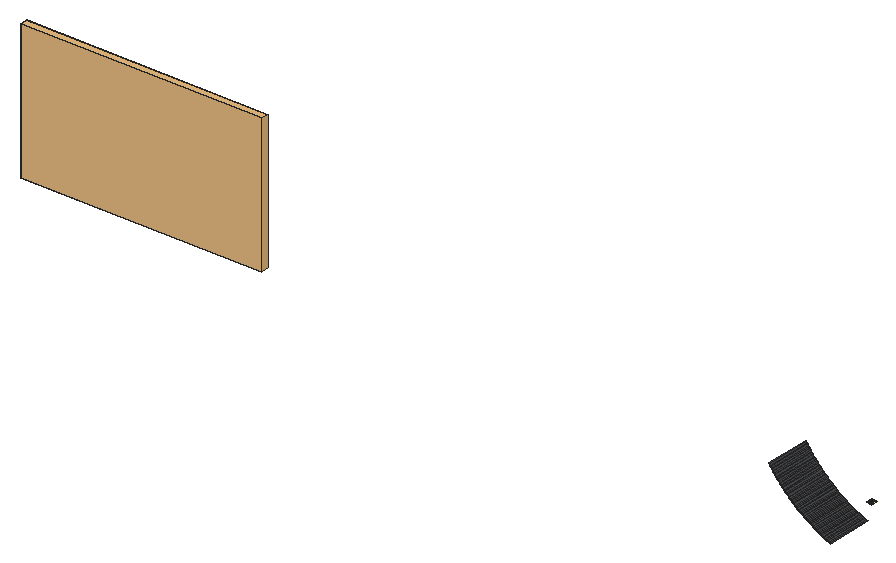
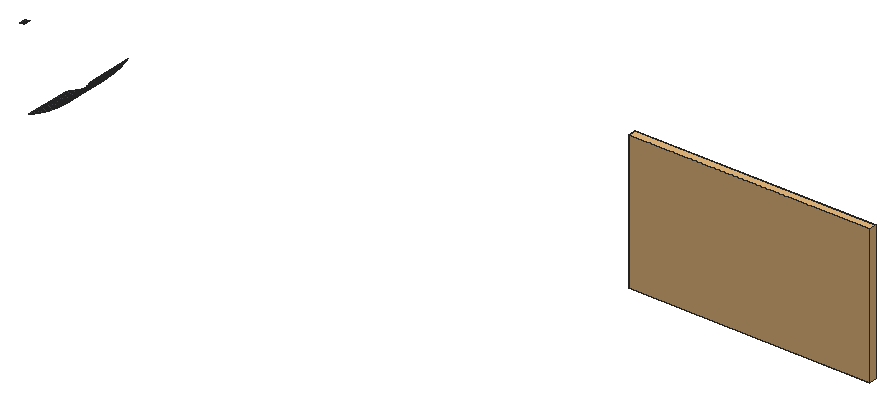
# SketchUp Ruby script. Lengths in inches.
U = 1.inch
M = Sketchup.active_model
def pt(a) = Geom::Point3d.new(a.map { |v| v * U })
def face(e, loops, mat)
  f = e.add_face(loops[0].map { |a| pt(a) })
  loops[1..].each { |l| e.add_face(l.map { |a| pt(a) }).erase! }
  f.material = f.back_material = mat if mat
  f
end
# faces: each face lists its corners as indices into pts; further lists are holes
def faces(e, pts, list, mat = nil) = list.each { |f| face(e, (f[0].is_a?(Array) ? f : [f]).map { |l| l.map { |i| pts[i] } }, mat) }
# xy, xz, yz: faces in a plane at the given z, y or x. An outline is a flat list of corners, or four numbers for a rectangle; further outlines are holes
def ring(l) = l.size == 4 ? [[l[0], l[1]], [l[2], l[1]], [l[2], l[3]], [l[0], l[3]]] : l.each_slice(2).to_a
def flat(e, list, mat, &to3) = list.each { |f| face(e, (f[0].is_a?(Array) ? f : [f]).map { |l| ring(l).map { |u, v| to3.(u, v) } }, mat) }
def xy(e, z, list, mat = nil) = flat(e, list, mat) { |x, y| [x, y, z] }
def xz(e, y, list, mat = nil) = flat(e, list, mat) { |x, z| [x, y, z] }
def yz(e, x, list, mat = nil) = flat(e, list, mat) { |y, z| [x, y, z] }
def lines(e, pts, list) = list.each { |a, b| e.add_line(pt(pts[a]), pt(pts[b])) }
# prism: a flat outline (further loops are holes) pulled along v
def prism(e, loops, v, mat = nil)
  f = face(e, loops, mat); d = Geom::Vector3d.new(v.map { |x| x * U })
  f.pushpull(f.normal.samedirection?(d) ? d.length : -d.length)
end
def box(e, o, s, mat = nil) = prism(e, [[o, [o[0] + s[0], o[1], o[2]], [o[0] + s[0], o[1] + s[1], o[2]], [o[0], o[1] + s[1], o[2]]]], [0, 0, s[2]], mat)
def at(x, y, z, deg = 0) = Geom::Transformation.translation(pt([x, y, z])) * Geom::Transformation.rotation(ORIGIN, Z_AXIS, deg.degrees)
def axes(o, x, y, z) = Geom::Transformation.new([*x, 0, *y, 0, *z, 0, *pt(o).to_a, 1])
def part(name) = M.definitions.add(name)
# library, detail: a bought-in or finely detailed component or shape, given as its bounding box
def library(name, o, s) = part(name).tap { |d| box(d.entities, o, s) }
def detail(e, o, s) = box(e.add_group.entities, o, s)
def put(e, d, t, mat = nil) = e.add_instance(d, t).tap { |i| i.material = mat if mat }
def group(e, t, mat = nil) = e.add_group.tap { |g| g.transformation = t; g.material = mat if mat }.entities
root = M.entities
M.materials.add("1432 AP 8245 TAR ROAD").color = [71, 72, 75]
M.materials.add("Outer Light").color = [251, 217, 152]
M.materials.add("[Wood Cherry Original]").color = [152, 86, 42]
c1 = library("Group\#43",[0,-2,0],[63,2,36])
p = [[264.96,107.37,158.64],[265.22,107.37,158.53],[265.22,95.37,158.53],[264.96,95.37,158.64],[264.7,107.37,158.75],[264.7,95.37,158.75],
  [264.44,107.37,158.87],[264.44,95.37,158.87],[264.19,107.37,158.98],[264.19,95.37,158.98],[263.93,107.37,159.1],[263.93,95.37,159.1],
  [263.67,107.37,159.22],[263.67,95.37,159.22],[263.42,107.37,159.34],[263.42,95.37,159.34],[263.16,107.37,159.46],[263.16,95.37,159.46],
  [262.91,107.37,159.59],[262.91,95.37,159.59],[262.66,107.37,159.72],[262.66,95.37,159.72],[262.4,107.37,159.85],[262.4,95.37,159.85],
  [262.15,107.37,159.98],[262.15,95.37,159.98],[261.91,107.37,160.11],[261.91,95.37,160.11],[261.66,107.37,160.25],[261.66,95.37,160.25],
  [261.41,107.37,160.38],[261.41,95.37,160.38],[261.16,107.37,160.52],[261.16,95.37,160.52],[260.92,107.37,160.66],[260.92,95.37,160.66],
  [260.67,107.37,160.81],[260.67,95.37,160.81],[260.43,107.37,160.95],[260.43,95.37,160.95],[260.19,107.37,161.1],[260.19,95.37,161.1],
  [259.95,107.37,161.25],[259.95,95.37,161.25],[259.71,107.37,161.4],[259.71,95.37,161.4],[259.47,107.37,161.55],[259.47,95.37,161.55],
  [259.24,107.37,161.7],[259.24,95.37,161.7],[259,107.37,161.86],[259,95.37,161.86],[258.76,107.37,162.02],[258.76,95.37,162.02],
  [258.53,107.37,162.18],[258.53,95.37,162.18],[258.3,107.37,162.34],[258.3,95.37,162.34],[258.07,107.37,162.5],[258.07,95.37,162.5],
  [257.84,107.37,162.67],[257.84,95.37,162.67],[257.61,107.37,162.83],[257.61,95.37,162.83],[257.38,107.37,163],[257.38,95.37,163],
  [257.16,107.37,163.17],[257.16,95.37,163.17],[256.94,107.37,163.35],[256.94,95.37,163.35],[256.71,107.37,163.52],[256.71,95.37,163.52],
  [256.49,107.37,163.7],[256.49,95.37,163.7],[256.27,107.37,163.875],[256.27,95.37,163.875],[256.05,107.37,164.05],[256.05,95.37,164.05],
  [255.84,107.37,164.23],[255.84,95.37,164.23],[255.62,107.37,164.42],[255.62,95.37,164.42],[255.41,107.37,164.6],[255.41,95.37,164.6],
  [255.19,107.37,164.79],[255.19,95.37,164.79],[254.98,107.37,164.98],[254.98,95.37,164.98],[254.77,107.37,165.17],[254.77,95.37,165.17],
  [254.5625,107.37,165.36],[254.5625,95.37,165.36],[254.36,107.37,165.55],[254.36,95.37,165.55],[254.15,107.37,165.74],[254.15,95.37,165.74],
  [253.95,107.37,165.94],[253.95,95.37,165.94],[253.74,107.37,166.14],[253.74,95.37,166.14],[253.54,107.37,166.34],[253.54,95.37,166.34],
  [253.35,107.37,166.54],[253.35,95.37,166.54],[253.15,107.37,166.74],[253.15,95.37,166.74],[252.95,107.37,166.94],[252.95,95.37,166.94],
  [252.76,107.37,167.15],[252.76,95.37,167.15],[252.5625,107.37,167.36],[252.5625,95.37,167.36],[252.375,107.37,167.5625],[252.375,95.37,167.5625],
  [252.18,107.37,167.77],[252.18,95.37,167.77],[252,107.37,167.98],[252,95.37,167.98],[251.81,107.37,168.2],[251.81,95.37,168.2],
  [251.625,107.37,168.41],[251.625,95.37,168.41],[251.44,107.37,168.63],[251.44,95.37,168.63],[251.26,107.37,168.84],[251.26,95.37,168.84],
  [251.08,107.37,169.0625],[251.08,95.37,169.0625],[250.9,107.37,169.28],[250.9,95.37,169.28],[250.73,107.37,169.5],[250.73,95.37,169.5],
  [250.55,107.37,169.73],[250.55,95.37,169.73],[250.38,107.37,169.95],[250.38,95.37,169.95],[250.21,107.37,170.18],[250.21,95.37,170.18],
  [250.04,107.37,170.4],[250.04,95.37,170.4],[249.875,107.37,170.63],[249.875,95.37,170.63],[249.71,107.37,170.86],[249.71,95.37,170.86],
  [249.55,107.37,171.09],[249.55,95.37,171.09],[249.38,107.37,171.32],[249.38,95.37,171.32],[249.23,107.37,171.56],[249.23,95.37,171.56],
  [275.63,95.37,171.57],[275.79,95.37,171.54],[275.79,96.87,171.54],[275.63,96.87,171.57],[275.63,96.87,171.57],[275.79,96.87,171.54],
  [275.79,95.37,171.54],[275.63,95.37,171.57],[275.95,95.37,171.52],[275.95,96.87,171.52],[275.95,96.87,171.52],[275.95,95.37,171.52],
  [249.07,107.37,171.79],[249.07,95.37,171.79],[275.16,95.37,171.66],[275.32,95.37,171.625],[275.32,96.87,171.625],[275.16,96.87,171.66],
  [275.16,96.87,171.66],[275.32,96.87,171.625],[275.32,95.37,171.625],[275.16,95.37,171.66],[275.48,95.37,171.6],[275.48,96.87,171.6],
  [275.48,96.87,171.6],[275.48,95.37,171.6],[274.69,95.37,171.75],[274.84,95.37,171.72],[274.84,96.87,171.72],[274.69,96.87,171.75],
  [274.69,96.87,171.75],[274.84,96.87,171.72],[274.84,95.37,171.72],[274.69,95.37,171.75],[275,95.37,171.6875],[275,96.87,171.6875],
  [275,96.87,171.6875],[275,95.37,171.6875]]
faces(root,p,[[0,1,2,3],[4,0,3,5],[6,4,5,7],[8,6,7,9],[10,8,9,11],[12,10,11,13],[14,12,13,15],[16,14,15,17],
  [18,16,17,19],[20,18,19,21],[22,20,21,23],[24,22,23,25],[26,24,25,27],[28,26,27,29],[30,28,29,31],[32,30,31,33],
  [34,32,33,35],[36,34,35,37],[38,36,37,39],[40,38,39,41],[42,40,41,43],[44,42,43,45],[46,44,45,47],[48,46,47,49],
  [50,48,49,51],[52,50,51,53],[54,52,53,55],[56,54,55,57],[58,56,57,59],[60,58,59,61],[62,60,61,63],[64,62,63,65],
  [66,64,65,67],[68,66,67,69],[70,68,69,71],[72,70,71,73],[74,72,73,75],[76,74,75,77],[78,76,77,79],[80,78,79,81],
  [82,80,81,83],[84,82,83,85],[86,84,85,87],[88,86,87,89],[90,88,89,91],[92,90,91,93],[94,92,93,95],[96,94,95,97],
  [98,96,97,99],[100,98,99,101],[102,100,101,103],[104,102,103,105],[106,104,105,107],[108,106,107,109],[110,108,109,111],[112,110,111,113],
  [114,112,113,115],[116,114,115,117],[118,116,117,119],[120,118,119,121],[122,120,121,123],[124,122,123,125],[126,124,125,127],[128,126,127,129],
  [130,128,129,131],[132,130,131,133],[134,132,133,135],[136,134,135,137],[138,136,137,139],[140,138,139,141],[142,140,141,143],[144,142,143,145],
  [146,144,145,147],[148,146,147,149],[150,151,152,153],[151,158,159,152],[162,148,149,163],[164,165,166,167],[165,172,173,166],[172,150,153,173],
  [176,177,178,179],[177,184,185,178],[184,164,167,185]],"1432 AP 8245 TAR ROAD")
faces(root,p,[[154,155,156,157],[155,160,161,156],[168,169,170,171],[169,174,175,170],[174,154,157,175],[180,181,182,183],[181,186,187,182],[186,168,171,187]],"Outer Light")
put(root,c1,at(51,100.37,167.79),"[Wood Cherry Original]")
